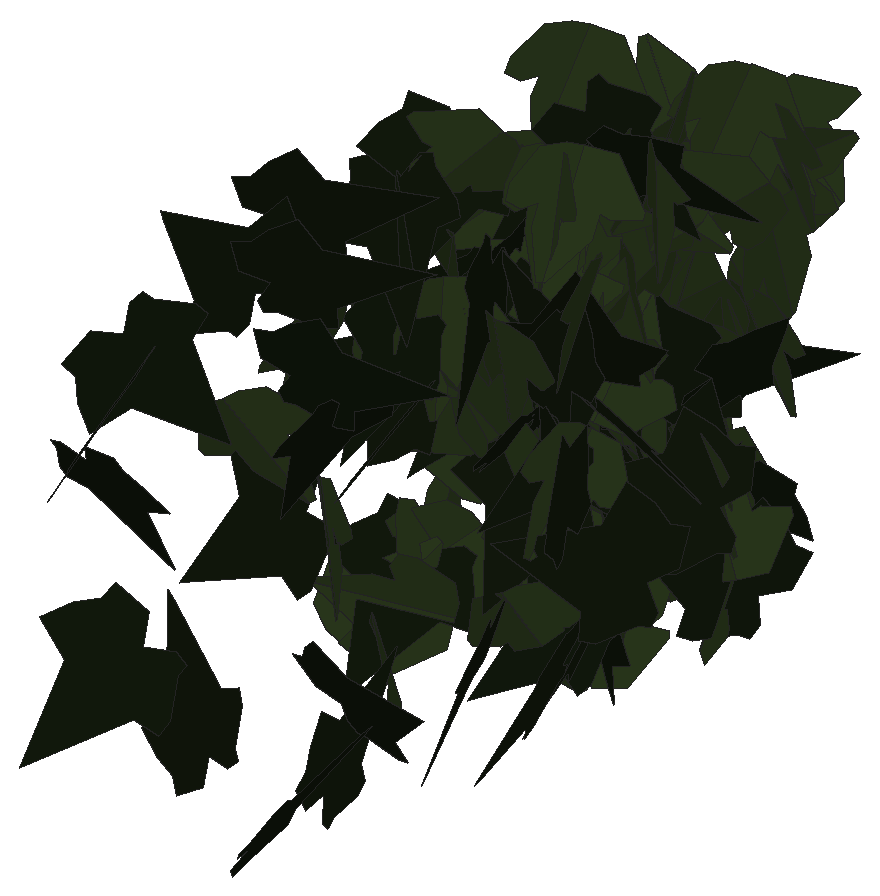
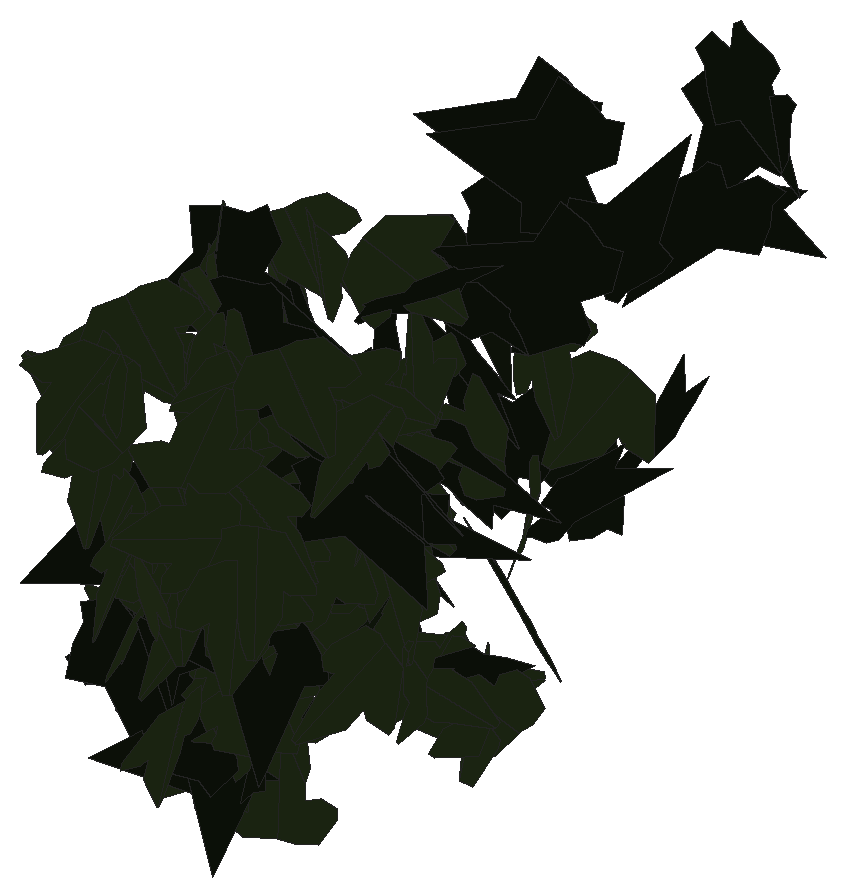
# SketchUp Ruby script. Lengths in inches.
U = 1.inch
M = Sketchup.active_model
def pt(a) = Geom::Point3d.new(a.map { |v| v * U })
def face(e, loops, mat)
  f = e.add_face(loops[0].map { |a| pt(a) })
  loops[1..].each { |l| e.add_face(l.map { |a| pt(a) }).erase! }
  f.material = f.back_material = mat if mat
  f
end
# faces: each face lists its corners as indices into pts; further lists are holes
def faces(e, pts, list, mat = nil) = list.each { |f| face(e, (f[0].is_a?(Array) ? f : [f]).map { |l| l.map { |i| pts[i] } }, mat) }
# xy, xz, yz: faces in a plane at the given z, y or x. An outline is a flat list of corners, or four numbers for a rectangle; further outlines are holes
def ring(l) = l.size == 4 ? [[l[0], l[1]], [l[2], l[1]], [l[2], l[3]], [l[0], l[3]]] : l.each_slice(2).to_a
def flat(e, list, mat, &to3) = list.each { |f| face(e, (f[0].is_a?(Array) ? f : [f]).map { |l| ring(l).map { |u, v| to3.(u, v) } }, mat) }
def xy(e, z, list, mat = nil) = flat(e, list, mat) { |x, y| [x, y, z] }
def xz(e, y, list, mat = nil) = flat(e, list, mat) { |x, z| [x, y, z] }
def yz(e, x, list, mat = nil) = flat(e, list, mat) { |y, z| [x, y, z] }
def lines(e, pts, list) = list.each { |a, b| e.add_line(pt(pts[a]), pt(pts[b])) }
# prism: a flat outline (further loops are holes) pulled along v
def prism(e, loops, v, mat = nil)
  f = face(e, loops, mat); d = Geom::Vector3d.new(v.map { |x| x * U })
  f.pushpull(f.normal.samedirection?(d) ? d.length : -d.length)
end
def box(e, o, s, mat = nil) = prism(e, [[o, [o[0] + s[0], o[1], o[2]], [o[0] + s[0], o[1] + s[1], o[2]], [o[0], o[1] + s[1], o[2]]]], [0, 0, s[2]], mat)
def at(x, y, z, deg = 0) = Geom::Transformation.translation(pt([x, y, z])) * Geom::Transformation.rotation(ORIGIN, Z_AXIS, deg.degrees)
def axes(o, x, y, z) = Geom::Transformation.new([*x, 0, *y, 0, *z, 0, *pt(o).to_a, 1])
def part(name) = M.definitions.add(name)
# library, detail: a bought-in or finely detailed component or shape, given as its bounding box
def library(name, o, s) = part(name).tap { |d| box(d.entities, o, s) }
def detail(e, o, s) = box(e.add_group.entities, o, s)
def put(e, d, t, mat = nil) = e.add_instance(d, t).tap { |i| i.material = mat if mat }
def group(e, t, mat = nil) = e.add_group.tap { |g| g.transformation = t; g.material = mat if mat }.entities
root = M.entities
M.materials.add("efeu1").color = [18, 25, 13]
M.materials.add("efeu2").color = [43, 57, 29]
c1 = part("ivyleaf_9")
p = [[1.54,2.16,1.25],[1.36,2.04,1.19],[-0.21,0.99,0.68],[-0.71,1.11,0.82],[-0.85,0.86,0.67],[-0.8,0.17,0.21],
  [-0.9,-0.01,0.1],[-0.67,-0.16,-0.02],[-0.08,-0.08,-0.05],[-0.03,-0.6,-0.4],[0.65,-0.88,-0.66],[0.83,-0.6,-0.49],
  [1.29,-0.42,-0.43],[1.8125,-0.07,-0.26],[1.21,0.44,0.15]]
faces(c1.entities,p,[[0,1,2,3,4,5,6,7,8,9,10,11,12,13,14]],"efeu1")
c2 = part("ivyleaf_10")
p = [[0,0.5,-0.03],[-0.0625,2.02,-0.43],[-0.19,2.01,-0.46],[-0.54,1.05,-0.29],[-0.52,0.625,-0.18],[-0.83,0.76,-0.28],
  [-1.16,0.64,-0.33],[-1.15,0.33,-0.24],[-0.77,-0.39,0.02],[-0.3,-0.51,0.16],[0.04,-0.48,0.23],[-0.02,2.01,-0.4375],
  [-0.06,2.01,-0.43],[0.04,-0.49,0.23],[0.67,-0.49,0.14],[1.38,0.36,-0.2],[1.375,0.51,-0.24],[0.81,0.65,-0.19],
  [0.62,0.59,-0.15],[0.6,1.09,-0.28],[0.5,1.23,-0.31]]
faces(c2.entities,p,[[0,1,2,3,4,5,6,7,8,9,10],[11,12,0,13,14,15,16,17,18,19,20]],"efeu2")
put(root,c1,axes([50.9,220.95,206.3],[0.09785,0.11952,0.47554],[-0.38369,-0.28326,0.15014],[0.3053,-0.39431,0.03629]))
put(root,c1,axes([50.51,221.87,206.51],[0.17695,-0.01575,0.46738],[0.46764,0.00869,-0.17675],[-0.00255,0.49968,0.0178]))
put(root,c1,axes([50.75,219.37,206.44],[0.02434,-0.21458,-0.45096],[-0.0069,0.4513,-0.21512],[0.49936,0.0167,0.01901]))
put(root,c2,axes([50.82,220.93,205],[-0.42073,-0.07857,-0.25847],[0.25359,0.05007,-0.428],[0.09314,-0.49124,-0.00228]))
put(root,c1,axes([51.08,221.41,203.89],[-0.21286,-0.27254,0.36112],[-0.18598,-0.31111,-0.34442],[0.41244,-0.28095,0.03107]))
put(root,c1,axes([51.48,222.56,204.83],[-0.21938,-0.0935,-0.43946],[-0.41285,-0.151,0.23823],[-0.17727,0.46739,-0.01095]))
put(root,c2,axes([50.83,222.56,202.22],[0.2893,0.18535,-0.36325],[0.31033,0.18888,0.34354],[0.26457,-0.42423,-0.00575]))
put(root,c2,axes([51.41,222.78,202.4],[-0.08361,-0.04745,-0.49067],[-0.46481,-0.15817,0.0945],[-0.16419,0.47194,-0.01766]))
put(root,c2,axes([51.13,221.58,205.78],[0.00866,-0.49988,0.00636],[0.00564,-0.00626,-0.49993],[0.49989,0.00873,0.00553]))
put(root,c2,axes([51,224.22,206.02],[0.02296,0.39368,0.3074],[0.02948,0.30612,-0.39424],[-0.4986,0.03623,-0.00916]))
put(root,c2,axes([51.03,224.25,203.48],[-0.10235,-0.24126,-0.42581],[0.18573,0.38334,-0.26184],[0.4528,-0.21177,0.01115]))
put(root,c1,axes([51.43,223.58,204.53],[-0.39267,-0.12337,0.28388],[-0.26969,-0.08868,-0.41158],[0.15191,-0.47636,0.0031]))
put(root,c2,axes([51.18,223.1,202.73],[0.01511,0.36203,-0.34454],[0.01701,0.34412,0.36234],[0.49948,-0.02267,-0.00192]))
put(root,c1,axes([51.2,223.05,202.79],[-0.33884,-0.36632,0.03163],[-0.02261,-0.02217,-0.499],[0.36699,-0.33959,-0.00154]))
put(root,c2,axes([51.22,225.19,206.98],[0.35799,0.3111,-0.1583],[-0.18061,-0.02895,-0.46534],[-0.2987,0.39036,0.09165]))
put(root,c2,axes([51.37,223.28,202.88],[0.27681,0.15357,-0.38703],[-0.35104,-0.16388,-0.31609],[-0.22393,0.44672,0.01709]))
put(root,c2,axes([51.3125,225.62,205.15],[-0.48885,-0.08687,0.05901],[-0.05264,-0.04043,-0.49558],[0.09087,-0.49073,0.03038]))
put(root,c1,axes([51.39,223.93,205.29],[0.12793,0.28214,-0.39247],[-0.15956,-0.35857,-0.30978],[-0.45626,0.20451,-0.0017]))
put(root,c2,axes([51.47,223.61,204.16],[-0.42533,-0.13629,0.22477],[-0.21418,-0.06815,-0.44663],[0.15238,-0.47621,-0.00041]))
put(root,c2,axes([51.42,224.15,206.13],[0.14428,0.19372,-0.43779],[-0.31142,-0.30929,-0.23949],[-0.36359,0.34178,0.0314]))
put(root,c2,axes([51.24,222.49,201.7],[-0.38095,0.29007,0.144],[0.10599,-0.0984,0.47863],[0.306,0.3952,0.01348]))
put(root,c1,axes([51.59,223.76,205.68],[-0.46394,0.17277,0.0701],[-0.06284,0.0321,-0.495],[-0.17554,-0.4681,-0.00807]))
put(root,c2,axes([51.6,223.32,204.98],[-0.3027,-0.20531,0.34091],[-0.27333,-0.20407,-0.36558],[0.28925,-0.40768,0.01131]))
put(root,c2,axes([50.96,222.59,205.03],[0.01161,-0.03998,0.49826],[0.49545,0.06698,-0.00617],[-0.06626,0.49388,0.04117]))
put(root,c2,axes([51.4,225.72,204.8],[-0.35478,-0.34999,-0.0405],[0.03681,0.02035,-0.49823],[0.3504,-0.3565,0.01133]))
put(root,c2,axes([51.25,221.58,203.96],[-0.18422,0.38303,-0.26335],[0.1128,-0.23797,-0.42502],[-0.45093,-0.216,0.00127]))
put(root,c1,axes([51.22,222.65,206.75],[-0.27625,-0.20396,-0.36344],[0.3631,0.09622,-0.33],[0.20455,-0.44626,0.09495]))
put(root,c1,axes([51.34,223.28,206.9],[-0.22222,-0.44205,0.07217],[0.04861,-0.10389,-0.48667],[0.44526,-0.20927,0.08915]))
put(root,c2,axes([51.29,223.1875,205.6875],[-0.37225,0.11884,0.31194],[0.27778,-0.14882,0.38819],[0.18511,0.46231,0.04477]))
put(root,c1,axes([51.63,223.69,204.69],[-0.49531,-0.04439,-0.05193],[0.05253,-0.00448,-0.49721],[0.04368,-0.49801,0.0091]))
put(root,c2,axes([51.57,225.57,204.73],[0.03252,0.35346,-0.35215],[-0.17979,-0.32089,-0.33868],[-0.46542,0.14865,0.10623]))
put(root,c2,axes([51.73,223.16,207.08],[-0.19341,-0.26503,0.37729],[-0.19028,-0.3268,-0.3271],[0.41998,-0.27011,0.02555]))
put(root,c1,axes([51.35,224.2,203.38],[0.1176,-0.43295,0.22074],[0.06214,-0.21185,-0.44862],[0.48198,0.13295,0.00398]))
put(root,c2,axes([51.87,224.04,205.59],[0.29436,0.00871,0.40408],[-0.40416,0.00334,0.29435],[0.00243,-0.49991,0.00901]))
put(root,c2,axes([51.28,223.34,203.91],[0.07283,0.01851,0.49432],[0.38476,0.31191,-0.06837],[-0.31089,0.39035,0.03119]))
put(root,c2,axes([51.76,222.94,204.7],[-0.11375,0.20435,0.44193],[-0.20762,0.39014,-0.23385],[-0.4404,-0.23671,-0.0039]))
put(root,c1,axes([51.84,217.85,206.85],[-0.28451,0.38313,-0.1492],[0.08895,-0.11979,-0.47722],[-0.40142,-0.29809,0]))
put(root,c1,axes([51.77,222.13,205.74],[-0.46911,-0.00886,-0.17279],[0.17236,0.01945,-0.46895],[0.01503,-0.49954,-0.0152]))
put(root,c2,axes([51.88,224.96,205.31],[0.39985,-0.06644,-0.29276],[-0.29038,0.03816,-0.40525],[0.07619,0.4941,-0.00807]))
put(root,c2,axes([51.875,223.05,204.39],[-0.32473,-0.24707,-0.28898],[-0.2258,-0.18043,0.40799],[-0.30589,0.39548,0.0056]))
put(root,c2,axes([51.8125,225.9,205.99],[0.30566,0.37632,0.12231],[-0.07699,-0.09504,0.48481],[0.38813,-0.3152,-0.00015]))
put(root,c1,axes([51.59,223.76,205.64],[0.09679,0.46909,0.14349],[-0.05033,-0.13599,0.47851],[0.48795,-0.10708,0.02089]))
put(root,c2,axes([51.73,222.63,205.68],[0.15646,0.46529,-0.095],[-0.03697,-0.08779,-0.49084],[-0.47345,0.16062,0.00693]))
put(root,c1,axes([51.97,224.57,203.64],[0.06081,0.49606,-0.01491],[-0.0019,-0.01479,-0.49978],[-0.49628,0.06084,0.00009]))
put(root,c2,axes([51.73,225.74,205.24],[-0.00592,-0.13661,0.48094],[0.10279,0.47037,0.13487],[-0.48929,0.10046,0.02252]))
put(root,c2,axes([51.82,224.04,204.24],[-0.2865,-0.36236,-0.19134],[0.15705,0.11855,-0.45965],[0.37849,-0.32348,0.04589]))
put(root,c1,axes([51.75,217.6,206.29],[0.48093,0.07056,-0.11716],[-0.11597,-0.01662,-0.48608],[-0.07249,0.49472,0.00038]))
put(root,c2,axes([51.84,226.12,203.43],[-0.02051,0.49955,-0.00535],[0.00306,-0.00523,-0.49996],[-0.49957,-0.02055,-0.00284]))
put(root,c2,axes([52.28,223.27,203.83],[-0.11174,-0.02134,0.48689],[-0.48653,-0.02413,-0.11272],[0.02831,-0.49896,-0.01537]))
put(root,c1,axes([52.09,218.8125,202.99],[-0.12962,-0.38454,0.29211],[0.09018,0.27786,0.40579],[-0.47441,0.15788,-0.00268]))
put(root,c1,axes([51.58,220.46,206.84],[0.21731,-0.01481,0.45006],[0.45024,0.01594,-0.21687],[-0.00792,0.49953,0.02026]))
put(root,c2,axes([51.9375,223.75,205.38],[0.43054,0.23489,-0.09727],[0.08458,0.04808,0.49044],[0.23976,-0.43876,0.00167]))
put(root,c1,axes([51.92,223.13,204.02],[-0.05424,0.48212,-0.12092],[-0.01371,0.12015,0.48516],[0.49686,0.05594,0.00018]))
put(root,c2,axes([52.14,222.95,205.375],[-0.48817,0.07534,0.07758],[-0.07661,0.01223,-0.49395],[-0.07633,-0.49414,-0.0004]))
put(root,c2,axes([52.05,224.33,201.49],[0.44351,0.23037,0.015],[-0.01333,-0.00688,0.49977],[0.23047,-0.44371,0.00004]))
put(root,c1,axes([51.93,223.05,205.92],[-0.06173,0.06135,-0.49237],[0.40612,-0.2788,-0.08566],[-0.28505,-0.4105,-0.01541]))
put(root,c2,axes([52.18,223.65,203.18],[0.32345,0.29683,-0.23931],[-0.18268,-0.15481,-0.43893],[-0.33467,0.37138,0.0083]))
put(root,c2,axes([52.49,224.9,202.85],[-0.34577,0.05903,-0.35632],[-0.35696,0.01928,0.34958],[0.05501,0.49613,0.02881]))
put(root,c1,axes([52.11,220.5,201.85],[-0.25343,0.38888,0.18587],[0.09084,-0.16258,0.46402],[0.42133,0.26896,0.01175]))
put(root,c2,axes([52.27,224.35,204.6],[-0.42816,-0.25712,-0.02383],[0.02036,0.01238,-0.49943],[0.25741,-0.42865,-0.00013]))
put(root,c2,axes([52.3125,224.51,203.13],[-0.39029,-0.31217,0.01508],[-0.01165,-0.00958,-0.49977],[0.31231,-0.39046,0.0002]))
put(root,c2,axes([52.3,224.0625,202.35],[-0.10849,-0.48807,0.00422],[-0.00074,-0.00416,-0.49998],[0.48809,-0.10849,0.00018]))
put(root,c1,axes([52.18,223.51,203.68],[-0.20192,-0.43499,0.14146],[0.01741,-0.16183,-0.47277],[0.45708,-0.186,0.0805]))
put(root,c1,axes([51.93,224.46,206.87],[-0.03273,-0.0955,-0.4897],[0.36308,0.33204,-0.08902],[0.3422,-0.36143,0.04762]))
put(root,c2,axes([52.27,224.74,202.82],[-0.404,-0.27157,-0.11417],[0.09551,0.06255,-0.48679],[0.27868,-0.41514,0.00134]))
put(root,c2,axes([52.25,224.48,206.24],[0.02055,-0.0548,0.49656],[-0.04312,0.49493,0.0564],[-0.49771,-0.04514,0.01562]))
put(root,c1,axes([52.06,224.41,203.6875],[0.22593,-0.44555,-0.02108],[-0.01845,0.01428,-0.49946],[0.44567,0.22646,-0.00999]))
put(root,c2,axes([52.52,224.83,204.19],[-0.38639,-0.195,0.25035],[-0.22476,-0.11031,-0.4328],[0.22403,-0.447,-0.00241]))
put(root,c1,axes([52.4,224.66,202.5625],[0.04011,0.4979,0.02202],[0.01109,0.02119,-0.49943],[-0.49827,0.04055,-0.00935]))
put(root,c2,axes([52.63,225.37,205.03],[-0.30492,-0.01741,0.39588],[-0.39537,-0.0202,-0.30541],[0.02663,-0.49929,-0.00145]))
put(root,c2,axes([52.33,224.83,202.45],[0.21069,0.40766,-0.19855],[-0.12425,-0.15866,-0.45759],[-0.43609,0.24216,0.03445]))
put(root,c2,axes([52.37,225.34,205.38],[0.31623,-0.38647,-0.02537],[-0.01577,0.01988,-0.49936],[0.38698,0.31662,0.00038]))
put(root,c1,axes([52.51,217.3125,204.79],[-0.39459,-0.28254,0.12029],[-0.10029,-0.06655,-0.4853],[0.29024,-0.40711,-0.00415]))
put(root,c2,axes([52.36,224.83,205.41],[-0.00064,-0.11474,0.48666],[0.13209,-0.46941,-0.1105],[0.48224,0.12842,0.03091]))
put(root,c2,axes([52.27,224.25,204.27],[0.3897,0.2357,-0.20634],[0.17491,0.10951,0.45543],[0.25988,-0.42714,0.0029]))
put(root,c2,axes([52.59,225.25,204.51],[-0.46858,-0.12145,0.12523],[-0.12081,-0.03303,-0.48406],[0.12585,-0.4839,0.0016]))
put(root,c2,axes([52.4375,225.04,206.39],[0.02086,0.17439,-0.46814],[-0.07713,-0.4618,-0.17547],[-0.49357,0.07953,0.00764]))
put(root,c1,axes([52.4,225.08,204.28],[-0.34002,-0.28372,-0.23214],[0.17464,0.15302,-0.44282],[0.32231,-0.38222,-0.00497]))
put(root,c1,axes([52.625,220.07,206.07],[-0.11154,0.41559,-0.25464],[0.05667,-0.2484,-0.43022],[-0.48409,-0.12484,0.00831]))
put(root,c1,axes([52.29,224.75,202.54],[0.20543,0.45442,0.03602],[-0.03064,-0.02565,0.4984],[0.45482,-0.20698,0.01731]))
put(root,c1,axes([52.28,224.65,202.31],[0.32452,0.04886,0.37723],[0.27849,0.30725,-0.27937],[-0.2591,0.39142,0.1722]))
put(root,c2,axes([52.51,224.86,203.84],[-0.00451,0.34131,0.36536],[-0.01936,0.36498,-0.3412],[-0.4996,-0.01723,0.00992]))
put(root,c1,axes([52.79,220.54,205.66],[-0.18863,0.46206,0.03024],[-0.01204,0.02775,-0.49908],[-0.4629,-0.18901,0.00066]))
put(root,c2,axes([52.44,223.19,207.02],[0.44986,-0.17508,0.13028],[0.12387,-0.0409,-0.48268],[0.17967,0.46656,0.00658]))
put(root,c1,axes([52.62,222.12,202.85],[-0.27704,0.2256,-0.34979],[0.27201,-0.21993,-0.35727],[-0.31506,-0.38825,-0.00087]))
put(root,c1,axes([52.91,222.93,205.18],[0.00729,-0.01577,0.4997],[-0.30701,0.39428,0.01692],[-0.39458,-0.30707,-0.00393]))
put(root,c2,axes([52.55,225.61,204.58],[0.17785,-0.39389,0.25144],[0.11782,-0.22254,-0.43196],[0.4522,0.2129,0.01366]))
put(root,c2,axes([52.5,224.375,202.57],[0.03264,-0.1689,-0.46947],[0.06878,-0.46446,0.17188],[-0.49417,-0.0758,-0.00709]))
put(root,c1,axes([52.29,224.12,202.22],[0.21865,-0.21613,-0.39431],[0.43213,-0.02022,0.25071],[-0.12432,-0.45042,0.17795]))
put(root,c2,axes([52.32,224.42,205.32],[0.17314,-0.10725,0.45664],[0.42979,-0.15872,-0.20023],[0.1879,0.46185,0.03723]))
put(root,c2,axes([52.66,225.76,204.92],[-0.14111,0.42729,0.21797],[-0.07396,0.20511,-0.44996],[-0.47394,-0.15923,0.00532]))
put(root,c1,axes([52.41,224.59,204.77],[-0.11864,-0.13169,-0.46753],[0.29362,0.36394,-0.17702],[0.38693,-0.31655,-0.00902]))
put(root,c2,axes([52.58,222.64,202.9],[-0.42362,-0.13067,-0.23124],[0.21679,0.08137,-0.44315],[0.15344,-0.47572,-0.01229]))
put(root,c2,axes([52.34,224.71,206.17],[-0.15026,-0.01141,-0.47675],[0.46578,-0.11078,-0.14414],[-0.10234,-0.48744,0.04392]))
put(root,c1,axes([52.6,223.44,205.11],[0.46785,0.05926,0.16613],[-0.16558,-0.01472,0.47156],[0.06077,-0.49626,0.00585]))
put(root,c2,axes([52.77,224.37,206.55],[0.20449,-0.36012,0.28018],[-0.13862,0.24348,0.41413],[-0.43471,-0.24704,-0.00027]))
put(root,c1,axes([53.01,222.91,204.63],[-0.44837,0.2192,-0.03023],[0.02698,-0.01364,-0.49909],[-0.21962,-0.44918,0.0004]))
put(root,c2,axes([52.75,223.23,207.13],[0.33423,0.34119,-0.14792],[-0.09478,-0.11416,-0.47748],[-0.35959,0.34722,-0.01164]))
put(root,c1,axes([52.37,219.76,206.47],[0.25085,-0.03616,0.43101],[0.42528,-0.07015,-0.2534],[0.07879,0.49373,-0.00444]))
put(root,c1,axes([53.08,222.97,202.92],[-0.49521,0.05391,0.04317],[-0.0431,0.00298,-0.49813],[-0.05397,-0.49708,0.00169]))
put(root,c2,axes([52.89,225.39,207.0625],[0.3054,0.34995,-0.18512],[-0.18955,-0.07601,-0.45639],[-0.34757,0.34894,0.08624]))
put(root,c1,axes([52.86,218.56,202.41],[-0.10021,0.47005,-0.13787],[-0.02925,0.13473,0.48062],[0.48898,0.10439,0.0005]))
put(root,c1,axes([52.625,223.91,206.93],[0.44269,0.07123,0.22126],[0.21829,0.03612,-0.44838],[-0.07986,0.49358,0.00089]))
put(root,c1,axes([52.67,220.05,203.11],[0.05252,-0.19289,0.45829],[0.36807,-0.29477,-0.16625],[0.33432,0.35483,0.11103]))
put(root,c1,axes([53.16,225.04,203.46],[0.29129,0.20144,-0.35295],[-0.29263,-0.19735,-0.35414],[-0.28199,0.41288,0.00292]))
put(root,c2,axes([53.29,224.97,206.35],[-0.17555,-0.21927,0.41364],[-0.24825,-0.33095,-0.28079],[0.39693,-0.30396,0.00733]))
put(root,c1,axes([53.2,222.96,202.96],[-0.36094,0.26197,-0.22604],[0.18353,-0.13196,-0.44599],[-0.29333,-0.40492,-0.00089]))
put(root,c2,axes([53,225.74,206.63],[-0.42666,0.21657,-0.14514],[0.12851,-0.06748,-0.47847],[-0.22683,-0.44559,0.00192]))
put(root,c1,axes([52.69,223.63,204.59],[0.28744,-0.32604,0.24715],[0.24575,-0.10389,-0.42287],[0.32709,0.36456,0.10052]))
put(root,c2,axes([53.12,222.84,204.5625],[0.18024,0.36486,-0.2905],[-0.12837,-0.2606,-0.40695],[-0.44837,0.22128,-0.00027]))
put(root,c2,axes([52.86,225.89,206.04],[-0.27638,-0.1634,0.38329],[0.35012,0.15828,0.31994],[-0.22589,0.44525,0.02693]))
put(root,c2,axes([53.17,225.54,205.67],[0.04932,0.47168,0.1584],[-0.12455,0.16581,-0.45497],[-0.48172,0.00542,0.13385]))
put(root,c2,axes([52.98,225.85,206.63],[0.21021,0.36841,0.26473],[0.11955,0.23648,-0.42401],[-0.43763,0.24156,0.01133]))
put(root,c2,axes([53.12,222.94,206.28],[0.2264,-0.40378,0.18896],[0.09171,-0.16522,-0.46292],[0.43627,0.24426,-0.00075]))
put(root,c2,axes([53,224.54,203.83],[-0.33996,0.2435,-0.27411],[0.23004,-0.14941,-0.41804],[-0.2855,-0.41035,-0.01044]))
put(root,c1,axes([53.35,222.23,202.74],[-0.36743,0.28052,-0.19054],[0.13633,-0.13505,-0.46171],[-0.3105,-0.39124,0.02276]))
put(root,c1,axes([53.46,222.21,204.3],[-0.0411,0.11013,0.48599],[-0.18068,0.45116,-0.11751],[-0.4644,-0.18528,0.00271]))
put(root,c2,axes([53.13,225.32,204.95],[-0.43737,0.20455,-0.12987],[0.11452,-0.06167,-0.48279],[-0.21352,-0.45206,0.00709]))
put(root,c1,axes([53.51,224.24,203.58],[-0.23238,-0.00583,0.44268],[-0.41095,-0.18314,-0.21813],[0.16469,-0.46521,0.08033]))
put(root,c2,axes([53.15,223.93,207.04],[-0.12468,0.42155,-0.23822],[0.05586,-0.23182,-0.43947],[-0.48097,-0.1362,0.01071]))
put(root,c1,axes([53.09,224.83,204.49],[0.26903,0.23038,0.35291],[0.24586,0.25427,-0.35341],[-0.34231,0.36369,0.02353]))
put(root,c2,axes([53.18,224.97,203.61],[-0.14787,0.44578,-0.17152],[0.06532,-0.15899,-0.46953],[-0.47315,-0.16126,-0.01121]))
put(root,c2,axes([53.3,224.51,202.18],[0.31135,-0.38803,0.04995],[-0.0132,0.05338,0.49697],[-0.39101,-0.31078,0.023]))
put(root,c1,axes([53.64,224.625,202.58],[0.01297,0.00013,0.49983],[-0.47628,-0.15166,0.01239],[0.15161,-0.47644,-0.00381]))
put(root,c1,axes([53.67,223.01,203.42],[-0.10687,-0.03199,0.4874],[-0.44281,-0.20423,-0.1105],[0.20615,-0.45527,0.01532]))
put(root,c2,axes([53.5,224.5,203.01],[0.4477,0.10221,0.19779],[-0.19276,-0.04431,0.45922],[0.1114,-0.48743,-0.00026]))
